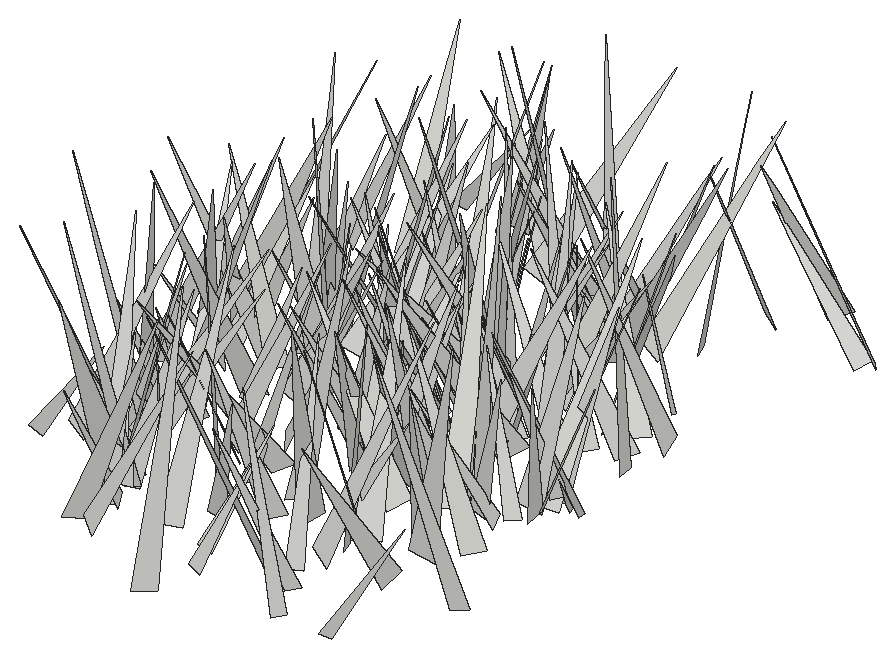
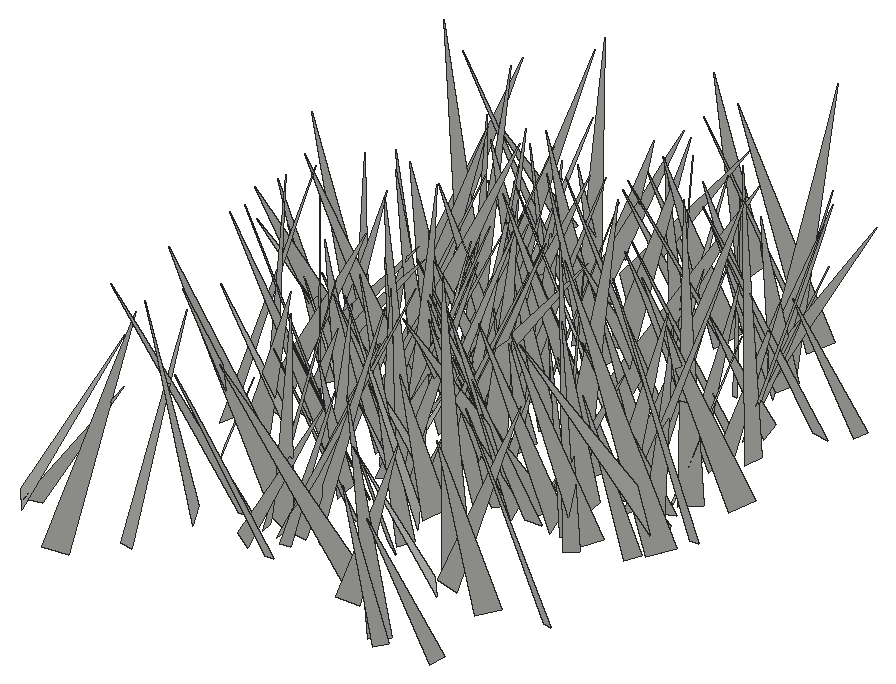
# SketchUp Ruby script. Lengths in inches.
U = 1.inch
M = Sketchup.active_model
def pt(a) = Geom::Point3d.new(a.map { |v| v * U })
def face(e, loops, mat)
  f = e.add_face(loops[0].map { |a| pt(a) })
  loops[1..].each { |l| e.add_face(l.map { |a| pt(a) }).erase! }
  f.material = f.back_material = mat if mat
  f
end
# faces: each face lists its corners as indices into pts; further lists are holes
def faces(e, pts, list, mat = nil) = list.each { |f| face(e, (f[0].is_a?(Array) ? f : [f]).map { |l| l.map { |i| pts[i] } }, mat) }
# xy, xz, yz: faces in a plane at the given z, y or x. An outline is a flat list of corners, or four numbers for a rectangle; further outlines are holes
def ring(l) = l.size == 4 ? [[l[0], l[1]], [l[2], l[1]], [l[2], l[3]], [l[0], l[3]]] : l.each_slice(2).to_a
def flat(e, list, mat, &to3) = list.each { |f| face(e, (f[0].is_a?(Array) ? f : [f]).map { |l| ring(l).map { |u, v| to3.(u, v) } }, mat) }
def xy(e, z, list, mat = nil) = flat(e, list, mat) { |x, y| [x, y, z] }
def xz(e, y, list, mat = nil) = flat(e, list, mat) { |x, z| [x, y, z] }
def yz(e, x, list, mat = nil) = flat(e, list, mat) { |y, z| [x, y, z] }
def lines(e, pts, list) = list.each { |a, b| e.add_line(pt(pts[a]), pt(pts[b])) }
# prism: a flat outline (further loops are holes) pulled along v
def prism(e, loops, v, mat = nil)
  f = face(e, loops, mat); d = Geom::Vector3d.new(v.map { |x| x * U })
  f.pushpull(f.normal.samedirection?(d) ? d.length : -d.length)
end
def box(e, o, s, mat = nil) = prism(e, [[o, [o[0] + s[0], o[1], o[2]], [o[0] + s[0], o[1] + s[1], o[2]], [o[0], o[1] + s[1], o[2]]]], [0, 0, s[2]], mat)
def at(x, y, z, deg = 0) = Geom::Transformation.translation(pt([x, y, z])) * Geom::Transformation.rotation(ORIGIN, Z_AXIS, deg.degrees)
def axes(o, x, y, z) = Geom::Transformation.new([*x, 0, *y, 0, *z, 0, *pt(o).to_a, 1])
def part(name) = M.definitions.add(name)
# library, detail: a bought-in or finely detailed component or shape, given as its bounding box
def library(name, o, s) = part(name).tap { |d| box(d.entities, o, s) }
def detail(e, o, s) = box(e.add_group.entities, o, s)
def put(e, d, t, mat = nil) = e.add_instance(d, t).tap { |i| i.material = mat if mat }
def group(e, t, mat = nil) = e.add_group.tap { |g| g.transformation = t; g.material = mat if mat }.entities
root = M.entities
c1 = part("fur_instance\#9")
p = [[0.8125,0,1.79],[0.67,-0.02,1.48],[0,-0.11,0],[0,0.11,0]]
faces(c1.entities,p,[[0,1,2,3]])
put(root,c1,axes([503.62,179.94,-21.66],[-7.70081,-2.50661,0.76749],[-2.60656,7.57519,-1.4131],[0.27927,1.58364,7.97425]))
put(root,c1,axes([498.68,176.65,-21.66],[1.93678,-3.59499,0.72466],[-3.24209,-1.29543,2.2385],[1.71404,1.61186,3.41529]))
put(root,c1,axes([498.39,191.1,-21.66],[4.54413,5.8348,1.67226],[5.93472,-3.83302,-2.75273],[1.27295,-2.95864,6.86415]))
put(root,c1,axes([498.81,202.99,-21.66],[3.86219,5.07234,0.99731],[5.04282,-3.42294,-2.11973],[1.1372,-2.04809,6.01264]))
put(root,c1,axes([498.79,186.54,-21.66],[5.79439,-3.93356,1.43708],[-4.17619,-5.2444,2.48372],[0.31237,2.85246,6.54821]))
put(root,c1,axes([503.06,190.74,-21.66],[-7.42684,-1.75978,1.28146],[-1.36577,7.3143,2.12899],[1.69519,-1.81689,7.32954]))
put(root,c1,axes([499.76,191.74,-21.66],[7.75154,3.11882,0.30174],[2.75499,-7.16733,3.30818],[-1.4927,2.96765,7.67264]))
put(root,c1,axes([501.88,188.59,-21.66],[-3.67716,-3.23058,0.06887],[-2.92053,3.36739,2.02339],[1.38271,-1.47883,4.45691]))
put(root,c1,axes([499.84,194.46,-21.66],[2.80159,-3.67069,0.58517],[-3.61323,-2.51742,1.50747],[0.87232,1.36159,4.36468]))
put(root,c1,axes([500.91,191.38,-21.66],[4.81338,-2.70132,0.36004],[-2.51999,-4.69011,-1.49931],[-1.0375,-1.14068,5.31205]))
put(root,c1,axes([505.99,176.46,-21.66],[-4.67528,-5.85921,0.505],[-5.43274,4.05599,-3.23694],[-2.25181,2.37953,6.76097]))
put(root,c1,axes([502.14,203.79,-21.66],[-4.09876,5.0884,1.14662],[4.86258,4.25523,-1.50159],[1.8873,0.0873,6.359]))
put(root,c1,axes([502.75,183.11,-21.66],[3.29812,-3.00828,0.87507],[-2.53709,-3.30998,-1.81667],[-1.83812,-0.82908,4.07763]))
put(root,c1,axes([503.48,183.9375,-21.66],[-5.02723,4.35262,0.08247],[4.19421,4.87628,-1.68986],[1.1665,1.22544,6.43138]))
put(root,c1,axes([499.05,193.05,-21.66],[3.50419,-7.42751,1.71848],[-7.22357,-2.63012,3.36199],[2.43745,2.88357,7.49295]))
put(root,c1,axes([504.45,189.89,-21.66],[0.94645,-5.69848,3.07489],[-6.04954,-1.88624,-1.63358],[-2.30884,2.60631,5.54074]))
put(root,c1,axes([500.32,178,-21.66],[3.27574,7.01328,0.4286],[6.91428,-3.13335,-1.57325],[1.25002,-1.04703,7.57902]))
put(root,c1,axes([501.39,182.36,-21.66],[7.9282,0.66664,2.15118],[1.11346,-8.00329,-1.62351],[-1.9576,-1.85234,7.78877]))
put(root,c1,axes([502.67,179.33,-21.66],[4.59265,0.40937,1.72839],[-0.43371,-4.3881,2.19176],[-1.72245,2.19644,4.05662]))
put(root,c1,axes([501.33,189.63,-21.66],[0.65579,5.75921,0.77226],[5.58682,-0.41126,-1.67728],[1.5976,-0.92592,5.54845]))
put(root,c1,axes([500.93,188.16,-21.66],[8.00988,-2.00577,0.3429],[-1.833,-7.71682,-2.32157],[-0.88363,-2.17404,7.92412]))
put(root,c1,axes([506.38,175.1875,-21.66],[-3.06653,-6.21678,2.70439],[-6.51984,1.89062,-3.04678],[-1.85842,3.62531,6.22648]))
put(root,c1,axes([504.77,192.14,-21.66],[-7.79963,1.89477,1.60693],[1.33324,7.65978,-2.56065],[2.09639,2.17814,7.60707]))
put(root,c1,axes([501.02,209.52,-21.66],[2.58418,-3.37784,0.00054],[-2.92311,-2.23595,2.1316],[1.69269,1.29557,3.68023]))
put(root,c1,axes([504.68,177.86,-21.66],[-4.29176,-1.39668,0.34406],[-1.22552,4.11722,1.42648],[0.75311,-1.25938,4.28195]))
put(root,c1,axes([504.99,175.16,-21.66],[-6.13848,3.83375,0.83292],[3.60337,6.1212,-1.61832],[1.55148,0.95163,7.05405]))
put(root,c1,axes([505.22,186.96,-21.66],[0.76231,-8.24421,0.75454],[-8.09051,-0.90251,-1.68715],[-1.75496,0.57958,8.10565]))
put(root,c1,axes([505.65,202.91,-21.66],[-0.4063,-5.76079,1.26429],[-5.69006,0.04941,-1.60344],[-1.5519,1.32705,5.54804]))
put(root,c1,axes([502.75,183.64,-21.66],[7.28027,0.47928,1.68125],[-0.05604,-7.13268,2.27604],[-1.74733,2.22571,6.93193]))
put(root,c1,axes([502.5625,194.63,-21.66],[4.48664,-4.30175,1.96808],[-4.72578,-3.95369,2.13158],[0.21294,2.89338,5.83878]))
put(root,c1,axes([504.76,182.91,-21.66],[3.23703,-3.40023,0.62778],[-3.13183,-3.24768,-1.44163],[-1.46538,-0.57015,4.46784]))
put(root,c1,axes([503.9375,194.95,-21.66],[-0.90647,-5.11686,1.80724],[-5.12934,1.40604,1.40817],[1.7715,1.45288,5.00209]))
put(root,c1,axes([502.8125,195.95,-21.66],[-1.84089,-7.99139,1.4242],[-7.16502,2.28604,3.56596],[3.81486,0.4373,7.3848]))
put(root,c1,axes([505.3,175.57,-21.66],[5.32876,3.34285,1.26399],[2.90072,-5.37113,1.97605],[-2.08763,1.0697,5.97207]))
put(root,c1,axes([507.53,191.28,-21.66],[-0.92246,-4.02488,0.49642],[-3.83236,0.69867,-1.45667],[-1.32631,0.78053,3.86377]))
put(root,c1,axes([505.39,193.96,-21.66],[-6.44163,0.17845,3.84936],[-1.24896,6.99677,-2.4144],[3.64548,2.71245,5.9747]))
put(root,c1,axes([506.64,172.82,-21.66],[-4.46885,1.59045,1.08144],[1.18804,4.43404,-1.61169],[1.51249,1.21632,4.46123]))
put(root,c1,axes([504.375,210.14,-21.66],[1.31964,-4.20384,0.49444],[-3.9297,-1.02429,1.77946],[1.57296,0.96785,4.03079]))
put(root,c1,axes([505.61,174.99,-21.66],[5.60712,-6.07402,0.33398],[-5.83929,-5.5015,-2.02021],[-1.70529,-1.13347,8.01575]))
put(root,c1,axes([506.0625,203.37,-21.66],[4.52328,4.39752,0.22155],[4.10164,-4.32376,2.0806],[-1.60118,1.34692,5.95561]))
put(root,c1,axes([508.7,207.52,-21.66],[-2.86629,5.19134,1.30889],[5.27356,2.48156,1.70596],[-0.92348,-1.94182,5.67938]))
put(root,c1,axes([503.59,181.27,-21.66],[3.2036,5.15972,0.63397],[4.7617,-2.61371,-2.78969],[2.08586,-1.95793,5.39475]))
put(root,c1,axes([506.85,173.54,-21.66],[-4.18199,-2.55213,0.91155],[-1.98836,4.02848,2.15666],[1.84139,-1.44616,4.39901]))
put(root,c1,axes([508.52,189.32,-21.66],[-6.74078,-2.87477,2.26806],[-3.46071,6.55422,-1.97791],[1.19661,2.76122,7.05622]))
put(root,c1,axes([504.91,209.54,-21.66],[1.45023,-6.39796,1.08768],[-6.25164,-1.07813,1.99368],[1.74182,1.45734,6.24998]))
put(root,c1,axes([503.61,178.27,-21.66],[4.07618,6.66518,0.05677],[6.29765,-3.82934,-2.59208],[2.18344,-1.39809,7.37028]))
put(root,c1,axes([505.53,186.06,-21.66],[1.80806,-4.3936,1.6396],[-4.55829,-1.23367,1.72079],[1.10181,2.10605,4.4285]))
put(root,c1,axes([507.14,190.56,-21.66],[6.25935,-4.83068,2.00086],[-4.50057,-6.56633,-1.77386],[-2.66155,-0.25726,7.70509]))
put(root,c1,axes([509.26,194.08,-21.66],[-0.23432,4.6061,1.3303],[4.44797,-0.2882,1.78136],[-1.78924,-1.31967,4.25416]))
put(root,c1,axes([506.16,174.98,-21.66],[-3.15581,4.82371,2.67558],[4.59437,4.00448,-1.80054],[3.05265,-1.04019,5.47589]))
put(root,c1,axes([506.54,177.47,-21.66],[-2.8265,-4.26887,1.57231],[-3.66111,3.23328,2.19698],[2.70032,-0.08465,4.62446]))
put(root,c1,axes([506.16,201.47,-21.66],[2.3597,-7.64104,0.82634],[-7.58316,-2.17409,1.55097],[1.25061,1.23463,7.84527]))
put(root,c1,axes([506.36,194.74,-21.66],[2.2285,7.10603,0.93052],[7.02267,-1.97084,-1.76797],[1.42959,-1.39565,7.23438]))
put(root,c1,axes([507.85,194.33,-21.66],[6.46332,2.41268,1.62775],[2.03661,-6.58136,1.66821],[-2.07914,1.05343,6.69422]))
put(root,c1,axes([506.21,170.58,-21.66],[6.24865,-3.61776,1.18124],[-3.80474,-5.99015,1.78079],[-0.08657,2.13519,6.99733]))
put(root,c1,axes([508.51,181.24,-21.66],[-3.43446,-5.67079,0.15135],[-5.3482,3.29577,2.1239],[1.89143,-0.97791,6.28032]))
put(root,c1,axes([506.53,193.7,-21.66],[-2.61013,7.00123,1.33294],[6.01827,2.92557,-3.58165],[3.81765,0.17478,6.55758]))
put(root,c1,axes([511.47,181.61,-21.66],[2.28844,-6.77562,0.58153],[-5.77223,-2.2597,-3.61376],[-3.59563,-0.68473,6.17144]))
put(root,c1,axes([509.52,193.23,-21.66],[-3.94963,4.34285,0.40783],[4.0226,3.83915,-1.92507],[1.68683,1.01332,5.54563]))
put(root,c1,axes([509.48,191.86,-21.66],[4.83042,2.64277,1.00625],[2.0268,-4.62442,2.4159],[-1.97202,1.72053,4.9478]))
put(root,c1,axes([510.96,176.8125,-21.66],[-6.29577,-3.22015,2.48262],[-3.79064,6.30377,-1.43636],[1.47099,2.46225,6.92409]))
put(root,c1,axes([510.93,197.32,-21.66],[-5.92228,3.52878,0.304],[3.26745,5.67188,-2.1844],[1.36692,1.73077,6.53866]))
put(root,c1,axes([506.74,188.15,-21.66],[3.69144,-5.31541,0.62902],[-5.0613,-3.21782,2.51095],[1.74141,1.9152,5.96452]))
put(root,c1,axes([510.52,201.54,-21.66],[2.07794,4.44656,0.23399],[4.16362,-2.03187,1.63715],[-1.57826,0.49406,4.62704]))
put(root,c1,axes([507.19,170.38,-21.66],[4.17015,5.48726,0.52169],[5.30168,-3.81404,-2.26221],[1.50809,-1.76505,6.51019]))
put(root,c1,axes([510.56,173.02,-21.66],[-6.29891,4.40553,1.36932],[3.82289,6.28157,-2.62437],[2.58248,1.44677,7.22479]))
put(root,c1,axes([507.51,182.16,-21.66],[3.41975,6.53108,1.33927],[6.45057,-2.86091,-2.51965],[1.68487,-2.30293,6.92828]))
put(root,c1,axes([511.57,188.73,-21.66],[-4.67511,2.29396,0.21165],[2.12082,4.47274,-1.63107],[0.89953,1.37696,4.94555]))
put(root,c1,axes([507.37,187.62,-21.66],[1.82991,-7.19945,3.13467],[-7.38413,-0.48301,3.20126],[2.67073,3.59742,6.70317]))
put(root,c1,axes([509.65,194.69,-21.66],[-4.5359,3.17744,2.60533],[2.766,5.23085,-1.56386],[3.0386,-0.01843,5.3127]))
put(root,c1,axes([512.42,195.79,-21.66],[-0.71726,5.0627,1.58469],[5.02661,0.13746,1.836],[-1.69568,-1.73401,4.77227]))
put(root,c1,axes([508.78,194.54,-21.66],[0.50211,5.33526,1.29674],[5.04367,0.06639,-2.22613],[2.16978,-1.38897,4.87457]))
put(root,c1,axes([509.16,191.11,-21.66],[3.22787,2.03353,0.24614],[1.96333,-2.94045,-1.45397],[0.58408,-1.35405,3.52709]))
put(root,c1,axes([510.95,179.24,-21.66],[5.49101,0.89671,2.25711],[-0.37206,-5.20349,2.97239],[-2.40004,2.85822,4.70322]))
put(root,c1,axes([511.35,198.18,-21.66],[6.37842,4.90538,1.53696],[4.59516,-6.53882,1.79932],[-2.30422,0.53885,7.84279]))
put(root,c1,axes([513.98,196.89,-21.66],[-4.11377,-6.51171,1.45116],[-6.65439,3.88319,-1.43913],[-0.47668,1.98739,7.56666]))
put(root,c1,axes([509.05,206.03,-21.66],[-0.59602,7.49567,1.64856],[6.68012,1.32078,-3.59019],[3.77872,-1.15261,6.60687]))
put(root,c1,axes([514.71,202.73,-21.66],[-5.12266,-6.1706,2.10185],[-6.50165,4.64284,-2.21548],[-0.47189,3.01719,7.70776]))
put(root,c1,axes([509.48,194.14,-21.66],[2.07826,-5.21506,0.82935],[-4.82149,-1.51054,2.58366],[2.15357,1.65083,4.98405]))
put(root,c1,axes([510.92,192.7,-21.66],[6.38764,-4.10189,0.26345],[-3.90919,-6.21298,-1.95294],[-1.27011,-1.50671,7.33577]))
put(root,c1,axes([514.6,190.93,-21.66],[-6.87538,0.87455,0.95023],[1.06547,6.75006,1.49673],[0.72976,-1.61573,6.76724]))
put(root,c1,axes([517.27,189.43,-21.66],[-4.42248,-6.55022,0.11235],[-5.68971,3.77318,-3.9833],[-3.24733,2.30957,6.8262]))
put(root,c1,axes([513.23,195.89,-21.66],[-6.54697,-3.05595,0.68846],[-2.14459,5.53525,4.1758],[2.28332,-3.56338,5.89613]))
put(root,c1,axes([509.73,183.95,-21.66],[5.9079,4.20697,0.32991],[4.15488,-5.69984,-1.72033],[0.73785,-1.5887,7.04573]))
put(root,c1,axes([510.15,200.8125,-21.66],[7.393,0.04175,0.28729],[0.1077,-7.1937,-1.72622],[-0.26959,-1.72907,7.18877]))
put(root,c1,axes([513.57,185.375,-21.66],[-5.24067,-3.21189,0.67738],[-2.84495,5.08085,2.08111],[1.63749,-1.45206,5.78359]))
put(root,c1,axes([513.97,166.71,-21.66],[-7.73799,2.57835,1.8542],[1.9672,7.72518,-2.53263],[2.4932,1.90688,7.75308]))
put(root,c1,axes([515.98,203.86,-21.66],[-8.04638,-2.10125,0.20494],[-2.02323,7.90531,1.61682],[0.60315,-1.51404,8.15753]))
put(root,c1,axes([512.46,195.23,-21.66],[4.4552,2.25801,0.37031],[2.04407,-4.29173,1.57715],[-1.02836,1.2518,4.7392]))
put(root,c1,axes([512.44,189.29,-21.66],[-0.90144,4.87523,0.09791],[4.65666,0.89022,-1.45364],[1.44671,0.1723,4.73998]))
put(root,c1,axes([515.92,193.46,-21.66],[-4.47703,-2.46915,0.00102],[-2.34184,4.24552,-1.62229],[-0.78262,1.42103,4.84857]))
put(root,c1,axes([511.85,186.57,-21.66],[0.68635,-5.64905,2.27441],[-5.90756,-0.06201,1.6287],[1.47832,2.3749,5.45254]))
put(root,c1,axes([513.93,196.61,-21.66],[3.59429,3.23742,0.8797],[2.57384,-3.488,2.32011],[-2.15177,1.23558,4.24464]))
put(root,c1,axes([511.96,175.37,-21.66],[0.90872,-5.0896,0.45336],[-4.90772,-0.74115,1.51668],[1.42262,0.69427,4.94262]))
put(root,c1,axes([514.4375,177.18,-21.66],[2.95346,-5.37759,1.21149],[-5.08452,-3.18852,-1.75785],[-2.12927,0.1548,5.87804]))
put(root,c1,axes([518.46,171.99,-21.66],[-5.00631,-5.98003,0.73957],[-5.22244,3.82659,-4.41068],[-3.00563,3.31169,6.43193]))
put(root,c1,axes([514.14,180.09,-21.66],[-6.72177,-1.11045,3.37602],[-2.29516,6.87097,-2.30972],[2.71346,3.06096,6.4094]))
put(root,c1,axes([515.55,195.58,-21.66],[1.80048,6.74236,1.9451],[6.61582,-2.30046,1.85022],[-2.33959,-1.31645,6.72888]))
put(root,c1,axes([515.43,203.5625,-21.66],[1.43774,-5.64122,0.58152],[-5.34924,-1.54822,-1.79367],[-1.88339,0.09091,5.53834]))
put(root,c1,axes([514.48,195.45,-21.66],[3.32895,2.2471,0.95718],[1.81279,-3.35751,1.57751],[-1.63691,0.85163,3.69362]))
put(root,c1,axes([514.99,185.49,-21.66],[-6.3203,-1.31951,1.76492],[-0.3807,5.93404,3.07318],[2.17051,-2.80147,5.67828]))
put(root,c1,axes([513.97,191.66,-21.66],[-3.49524,-7.20934,0.56433],[-6.86604,3.50524,2.25399],[2.26947,-0.49846,7.68835]))
put(root,c1,axes([516.31,203.49,-21.66],[1.43872,7.93621,2.15807],[7.82752,-1.99366,2.11323],[-2.52399,-1.65906,7.7838]))
put(root,c1,axes([515.67,195.96,-21.66],[-6.83742,-2.67371,1.15288],[-1.91772,6.34944,3.35188],[2.19094,-2.7864,6.53176]))
put(root,c1,axes([514.07,179.59,-21.66],[6.87844,-2.02965,2.77665],[-2.6588,-7.07628,1.41394],[-2.18175,2.22463,7.03088]))
put(root,c1,axes([515.23,188.3125,-21.66],[2.94915,-5.28887,0.70098],[-5.06545,-3.02722,-1.5291],[-1.67475,-0.15728,5.85931]))
put(root,c1,axes([512.29,189.17,-21.66],[3.25743,4.86298,0.41292],[4.6269,-2.91916,-2.12138],[1.55271,-1.50328,5.4552]))
put(root,c1,axes([517.1875,205.8,-21.66],[-2.08811,-4.65792,0.59921],[-4.45757,1.75934,-1.85749],[-1.47829,1.27435,4.7546]))
put(root,c1,axes([517.51,188.95,-21.66],[-4.9951,-5.23204,0.99068],[-5.30492,4.77148,-1.54841],[-0.46216,1.77916,7.06595]))
put(root,c1,axes([513.07,196.98,-21.66],[1.49707,-8.01218,1.60299],[-8.01526,-1.12338,1.87068],[1.58751,1.88383,7.93327]))
put(root,c1,axes([513.62,172.28,-21.66],[-0.24087,4.17753,0.95098],[3.88217,0.61574,-1.72155],[1.81241,-0.76371,3.81393]))
put(root,c1,axes([515.04,204.85,-21.66],[3.98276,-1.20965,1.22676],[-0.42908,-3.68899,-2.24451],[-1.66855,-1.93873,3.5054]))
put(root,c1,axes([516.61,192.07,-21.66],[0.00954,3.59248,1.3323],[3.47361,-0.5704,1.51319],[-1.6171,-1.20405,3.25826]))
put(root,c1,axes([516.06,194,-21.66],[-6.64988,-1.58039,2.79885],[-2.32051,6.81074,-1.66765],[2.22405,2.38079,6.62853]))
put(root,c1,axes([516.16,198.34,-21.66],[-5.21181,1.32812,1.31914],[0.83689,5.14396,-1.87252],[1.67442,1.56295,5.04188]))
put(root,c1,axes([513.8125,195.89,-21.66],[7.80685,-2.34529,0.78759],[-1.91376,-7.37702,-2.99744],[-1.56786,-2.67335,7.58041]))
put(root,c1,axes([514.33,184.54,-21.66],[6.011,-2.52803,0.45147],[-2.2406,-5.7244,-2.22212],[-1.25478,-1.8887,6.13068]))
put(root,c1,axes([518.03,197.1,-21.66],[-7.28792,0.99409,0.70676],[0.80322,7.1337,-1.75122],[0.9179,1.65037,7.1439]))
put(root,c1,axes([516.79,184.49,-21.66],[1.83922,3.08635,0.93557],[2.6886,-2.06216,1.51739],[-1.78108,0.07419,3.25666]))
put(root,c1,axes([518.72,182.31,-21.66],[-6.43604,2.78332,0.65453],[2.85741,6.20344,1.71766],[-0.1023,-1.83529,6.79846]))
put(root,c1,axes([513.81,200.45,-21.66],[2.98745,4.37857,0.43851],[4.21633,-2.69647,-1.80015],[1.25963,-1.35874,4.98559]))
put(root,c1,axes([514.57,170.16,-21.66],[0.74077,3.76285,1.03817],[3.63302,-0.27816,-1.5841],[1.42759,-1.24465,3.49262]))
put(root,c1,axes([515.92,184.47,-21.66],[4.34994,-4.04005,0.73934],[-3.73736,-4.34022,-1.72779],[-1.70317,-0.79441,5.67968]))
put(root,c1,axes([515.64,193.3,-21.66],[-3.26721,-5.06008,0.08616],[-4.54982,2.98181,2.58736],[2.21606,-1.33826,5.43917]))
put(root,c1,axes([518.61,185.84,-21.66],[-0.87207,-5.64239,2.10409],[-5.67136,0.05471,-2.20385],[-2.02471,2.277,5.26688]))
put(root,c1,axes([517.01,204.01,-21.66],[-6.19203,-3.31038,1.54754],[-2.85802,6.28451,2.00782],[2.2771,-1.114,6.72819]))
put(root,c1,axes([516.36,185.18,-21.66],[-3.94538,2.89092,1.6801],[2.22143,4.20848,-2.02488],[2.49909,0.82308,4.45234]))
put(root,c1,axes([514.875,198.07,-21.66],[3.37481,3.69249,0.11879],[3.55193,-3.19874,-1.47981],[1.01606,-1.08238,4.77849]))
put(root,c1,axes([518.82,190.21,-21.66],[-6.06549,-1.51995,0.44377],[-1.27134,5.72216,2.22212],[0.94386,-2.06007,5.84487]))
put(root,c1,axes([514.91,206.36,-21.66],[2.90433,5.023,0.38727],[4.82562,-2.64532,-1.87916],[1.44702,-1.25991,5.48948]))
put(root,c1,axes([518.74,173.42,-21.66],[0.42359,6.38348,0.10104],[6.1795,-0.43539,1.60081],[-1.60398,0.00839,6.194]))
put(root,c1,axes([520.38,193.49,-21.66],[-2.56552,5.11443,0.44811],[4.78646,2.20153,2.27666],[-1.85689,-1.39139,5.24939]))
put(root,c1,axes([519.24,191.86,-21.66],[-1.9475,3.70978,1.3462],[3.85912,1.47603,1.51527],[-0.82582,-1.85103,3.9063]))
put(root,c1,axes([516.14,178.07,-21.66],[7.64117,-3.1953,0.94942],[-2.87226,-7.51641,-2.18001],[-1.69158,-1.67105,7.9903]))
put(root,c1,axes([519.05,190.72,-21.66],[-4.78281,-0.5343,0.54387],[-0.29464,4.48183,1.81189],[0.70318,-1.75621,4.45846]))
put(root,c1,axes([516.04,184.54,-21.66],[0.11042,6.13884,2.00494],[6.14565,0.51615,-1.91884],[1.98398,-1.94051,5.83229]))
put(root,c1,axes([519.72,185.27,-21.66],[-6.83596,-2.73328,0.53057],[-2.58478,6.75268,1.48423],[1.035,-1.18879,7.21098]))
put(root,c1,axes([517.64,193.3125,-21.66],[5.12063,-0.00436,1.95562],[-0.62511,-5.19742,1.62522],[-1.85303,1.74129,4.85588]))
put(root,c1,axes([520,171.78,-21.66],[0.21984,-5.04241,1.33274],[-4.72838,-0.75562,-2.0789],[-2.20101,1.11963,4.59917]))
put(root,c1,axes([518.68,189.41,-21.66],[-3.83157,-3.11067,0.41222],[-2.87249,3.73899,1.51524],[1.26294,-0.9332,4.69694]))
put(root,c1,axes([519.47,186.56,-21.66],[1.15539,6.15443,1.22459],[6.01284,-1.44203,1.57415],[-1.79512,-0.86897,6.06086]))
put(root,c1,axes([521.23,168.98,-21.66],[0.1109,6.16383,0.84068],[5.38265,-0.51661,3.07768],[-3.11876,-0.67243,5.34163]))
put(root,c1,axes([520.01,190.46,-21.66],[4.91107,-6.51993,1.1851],[-5.42781,-4.80392,-3.93621],[-3.80168,-1.5638,7.15082]))
put(root,c1,axes([517.67,184.36,-21.66],[-0.91329,-6.82842,0.06821],[-6.63421,0.90353,1.6239],[1.61843,-0.14959,6.69511]))
put(root,c1,axes([519.76,178.24,-21.66],[-5.97227,4.9002,0.90124],[4.6479,5.98621,-1.7477],[1.79477,0.80344,7.52499]))
put(root,c1,axes([519.42,177.01,-21.66],[-5.36603,-1.88935,2.74168],[-2.67241,5.54565,-1.40882],[1.98613,2.35731,5.51173]))
put(root,c1,axes([521.15,191.73,-21.66],[-7.41355,2.38035,1.13819],[1.92535,7.2016,-2.52036],[1.80404,2.09598,7.36713]))
put(root,c1,axes([519.4375,190.64,-21.66],[5.08694,2.79276,1.06084],[2.31416,-5.00849,2.08845],[-1.88933,1.38471,5.41433]))
put(root,c1,axes([517.45,178.58,-21.66],[1.13497,4.33314,1.68645],[4.04549,-0.06445,-2.557],[2.29221,-2.03177,3.67778]))
put(root,c1,axes([521.26,183.85,-21.66],[-6.0602,5.67803,0.65626],[5.53411,6.06799,-1.39639],[1.4298,0.57987,8.18634]))
put(root,c1,axes([522.51,175.57,-21.66],[-5.08452,-4.09315,0.88657],[-4.17476,4.84247,-1.58557],[-0.33349,1.78573,6.33184]))
put(root,c1,axes([521.66,185.14,-21.66],[-7.99125,0.08509,2.25297],[-0.74491,7.73167,-2.93422],[2.12796,3.02611,7.43355]))
put(root,c1,axes([518.09,196.28,-21.66],[1.6055,7.88479,1.47704],[7.72527,-1.11383,-2.45126],[2.16141,-1.87581,7.66412]))
put(root,c1,axes([520.33,182.71,-21.66],[7.53052,-1.13144,2.64431],[-0.30654,-7.68469,-2.41514],[-2.85982,-2.15562,7.22191]))
put(root,c1,axes([522.91,193.3,-21.66],[-0.96186,4.58475,0.31518],[4.19254,0.74357,1.97843],[-1.88199,-0.68675,4.24628]))
put(root,c1,axes([520.75,205.32,-21.66],[6.22186,3.72093,2.03459],[3.43335,-6.54009,1.46143],[-2.48938,0.27987,7.10078]))
put(root,c1,axes([519.85,199.87,-21.66],[6.47636,2.00005,0.90058],[1.74291,-6.39683,1.67254],[-1.33173,1.35459,6.56857]))
put(root,c1,axes([517.88,201.39,-21.66],[7.15691,-3.14413,0.26361],[-3.09126,-6.8566,2.14652],[0.63178,2.06831,7.5166]))
put(root,c1,axes([518.65,203.6,-21.66],[2.72489,7.5123,0.23605],[7.26372,-2.56761,-2.13568],[1.931,-0.94238,7.70056]))
put(root,c1,axes([518.34,189.47,-21.66],[2.77972,-6.83526,2.99642],[-7.05556,-1.36449,3.4327],[2.43278,3.85274,6.53179]))
put(root,c1,axes([518.97,175.32,-21.66],[3.76818,7.24013,0.96766],[7.17608,-3.46602,-2.01138],[1.36373,-1.76699,7.91031]))
put(root,c1,axes([524.1,195.94,-21.66],[-2.5947,5.83184,0.30944],[5.66182,2.42897,1.69778],[-1.43174,-0.96349,6.15308]))
put(root,c1,axes([521.63,210.125,-21.66],[-2.90473,-5.90083,0.221],[-5.68544,2.86131,1.67173],[1.5951,-0.54696,6.36102]))
put(root,c1,axes([521.09,194.48,-21.66],[-4.22534,-4.50008,2.6097],[-4.33201,4.90527,1.44456],[2.88009,0.77613,6.00146]))
put(root,c1,axes([523.93,199.02,-21.66],[-3.59352,-1.36236,0.30323],[-1.35819,3.22059,-1.62619],[-0.32136,1.6227,3.48208]))
put(root,c1,axes([526.19,187.54,-21.66],[-4.35257,-4.39527,0.35538],[-3.69396,3.36161,-3.66659],[-2.40819,2.78761,4.98191]))
put(root,c1,axes([524.86,193.95,-21.66],[-3.6368,4.97548,2.15784],[5.29036,2.68314,2.72961],[-1.1932,-3.26854,5.52548]))
put(root,c1,axes([517.91,196.09,-21.66],[5.88193,4.68919,0.48239],[4.10623,-4.71789,-4.20698],[2.31519,-3.54559,6.23594]))
put(root,c1,axes([521.33,180.84,-21.66],[5.7747,-1.11479,0.95698],[-0.77258,-5.60537,-1.86777],[-1.24967,-1.68603,5.57685]))
put(root,c1,axes([523.875,184.11,-21.66],[-4.91943,-1.92287,0.32626],[-1.70701,4.67316,1.80343],[0.9434,-1.57124,4.96446]))
put(root,c1,axes([524.42,184.8125,-21.66],[-1.36293,4.52681,0.55653],[4.38086,1.13777,1.47406],[-1.26877,-0.93423,4.49185]))
put(root,c1,axes([522.22,195.23,-21.66],[4.78963,3.34115,0.62659],[3.09789,-4.73577,1.57225],[-1.39963,0.95165,5.62422]))
put(root,c1,axes([525.01,180.76,-21.66],[-3.75455,5.21199,1.89568],[5.51913,3.28609,1.89629],[-0.5456,-2.62523,6.13723]))
put(root,c1,axes([526.97,187.46,-21.66],[-3.79929,-4.93063,0.76728],[-4.2284,2.66909,-3.78564],[-2.64961,2.81057,4.94112]))
put(root,c1,axes([523.48,175.77,-21.66],[5.96418,-2.86813,1.57613],[-1.66285,-5.47776,-3.67572],[-2.81874,-2.83722,5.50334]))
put(root,c1,axes([524.2,212.9,-21.66],[4.00993,-5.51552,0.33203],[-5.14979,-3.87921,-2.24547],[-2.00271,-1.06842,6.43882]))
put(root,c1,axes([522.63,184.2,-21.66],[0.54307,-5.39112,1.14857],[-5.29865,-0.1925,1.60174],[1.51911,1.25582,5.17624]))
put(root,c1,axes([525.84,192.57,-21.66],[-7.59721,-1.99805,2.32928],[-2.54922,7.5713,-1.81993],[1.70857,2.41215,7.64184]))
put(root,c1,axes([522.48,190.7,-21.66],[4.18709,2.7222,0.51054],[2.74144,-3.94162,-1.4666],[0.39441,-1.502,4.77401]))
put(root,c1,axes([525.93,196.23,-21.66],[-7.13222,-2.21187,1.52983],[-1.72076,7.08542,2.22194],[2.06682,-1.73369,7.12909]))
put(root,c1,axes([525.35,187.8125,-21.66],[3.42862,-3.42654,1.21049],[-3.04602,-3.61734,-1.61199],[-1.98197,-0.36822,4.57144]))
put(root,c1,axes([523.2,178.74,-21.66],[1.45469,-7.67033,1.86376],[-7.74266,-1.0178,1.85445],[1.53584,2.13396,7.5836]))
put(root,c1,axes([524.87,186.86,-21.66],[-5.0261,5.87636,0.71878],[5.2638,4.86732,-2.98524],[2.70938,1.44485,7.13314]))
put(root,c1,axes([528.29,175.49,-21.66],[-0.67807,6.71445,3.30984],[6.96597,-0.65101,2.74773],[-2.74118,-3.31527,6.16389]))
put(root,c1,axes([525.05,186.42,-21.66],[5.40862,3.75774,0.29196],[3.28966,-4.95573,2.84217],[-1.83956,2.18614,5.94103]))
put(root,c1,axes([524.01,189.29,-21.66],[3.16186,-4.77933,2.12939],[-5.21892,-2.70344,1.68164],[0.37303,2.68757,5.47827]))
put(root,c1,axes([528.46,209.41,-21.66],[-4.24155,2.82864,0.08548],[2.61337,3.85608,2.07369],[-1.08573,-1.76881,4.65744]))
put(root,c1,axes([529.08,209.7,-21.66],[-5.24888,-4.54366,0.15791],[-4.36596,4.97023,-2.11085],[-1.26815,1.69482,6.61361]))
put(root,c1,axes([524.28,186.36,-21.66],[1.86303,-6.4471,2.90273],[-6.99316,-1.23765,1.73947],[1.04242,3.21946,6.48153]))
put(root,c1,axes([525.15,185.78,-21.66],[5.21183,-0.69159,1.00189],[-0.40075,-5.13378,-1.45906],[-1.14955,-1.3458,5.051]))
put(root,c1,axes([524.48,168.87,-21.66],[3.53802,-1.77872,0.68161],[-1.86523,-2.94336,2.00089],[0.38644,2.07817,3.41729]))
